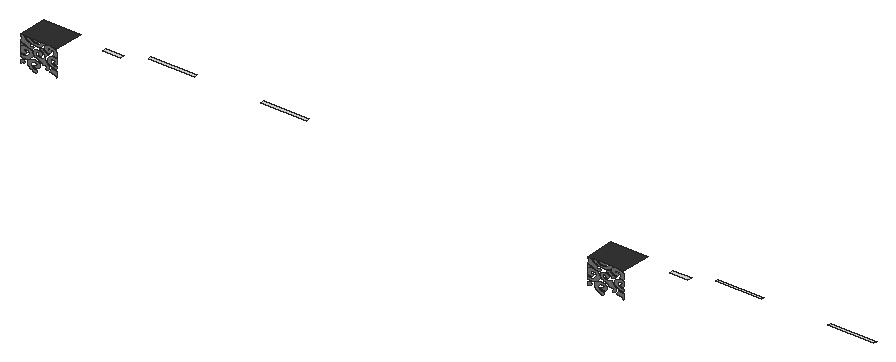
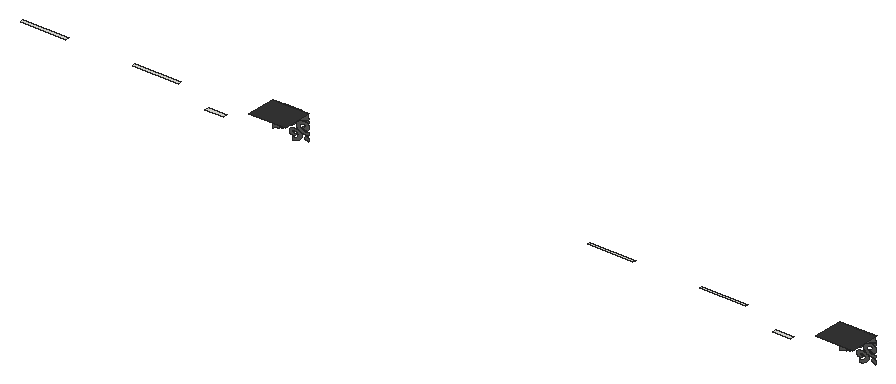
# SketchUp Ruby script. Lengths in inches.
U = 1.inch
M = Sketchup.active_model
def pt(a) = Geom::Point3d.new(a.map { |v| v * U })
def face(e, loops, mat)
  f = e.add_face(loops[0].map { |a| pt(a) })
  loops[1..].each { |l| e.add_face(l.map { |a| pt(a) }).erase! }
  f.material = f.back_material = mat if mat
  f
end
# faces: each face lists its corners as indices into pts; further lists are holes
def faces(e, pts, list, mat = nil) = list.each { |f| face(e, (f[0].is_a?(Array) ? f : [f]).map { |l| l.map { |i| pts[i] } }, mat) }
# xy, xz, yz: faces in a plane at the given z, y or x. An outline is a flat list of corners, or four numbers for a rectangle; further outlines are holes
def ring(l) = l.size == 4 ? [[l[0], l[1]], [l[2], l[1]], [l[2], l[3]], [l[0], l[3]]] : l.each_slice(2).to_a
def flat(e, list, mat, &to3) = list.each { |f| face(e, (f[0].is_a?(Array) ? f : [f]).map { |l| ring(l).map { |u, v| to3.(u, v) } }, mat) }
def xy(e, z, list, mat = nil) = flat(e, list, mat) { |x, y| [x, y, z] }
def xz(e, y, list, mat = nil) = flat(e, list, mat) { |x, z| [x, y, z] }
def yz(e, x, list, mat = nil) = flat(e, list, mat) { |y, z| [x, y, z] }
def lines(e, pts, list) = list.each { |a, b| e.add_line(pt(pts[a]), pt(pts[b])) }
# prism: a flat outline (further loops are holes) pulled along v
def prism(e, loops, v, mat = nil)
  f = face(e, loops, mat); d = Geom::Vector3d.new(v.map { |x| x * U })
  f.pushpull(f.normal.samedirection?(d) ? d.length : -d.length)
end
def box(e, o, s, mat = nil) = prism(e, [[o, [o[0] + s[0], o[1], o[2]], [o[0] + s[0], o[1] + s[1], o[2]], [o[0], o[1] + s[1], o[2]]]], [0, 0, s[2]], mat)
def at(x, y, z, deg = 0) = Geom::Transformation.translation(pt([x, y, z])) * Geom::Transformation.rotation(ORIGIN, Z_AXIS, deg.degrees)
def axes(o, x, y, z) = Geom::Transformation.new([*x, 0, *y, 0, *z, 0, *pt(o).to_a, 1])
def part(name) = M.definitions.add(name)
# library, detail: a bought-in or finely detailed component or shape, given as its bounding box
def library(name, o, s) = part(name).tap { |d| box(d.entities, o, s) }
def detail(e, o, s) = box(e.add_group.entities, o, s)
def put(e, d, t, mat = nil) = e.add_instance(d, t).tap { |i| i.material = mat if mat }
def group(e, t, mat = nil) = e.add_group.tap { |g| g.transformation = t; g.material = mat if mat }.entities
root = M.entities
M.materials.add("[0043_SaddleBrown]4").color = [124, 123, 122]
M.materials.add("[Slate Light Tile]").color = [54, 54, 54]
xy(root,742.22,[[2997.35,656.57,3037.18,665.86],[4247.98,656.57,4287.81,665.86]])
xy(root,759.44,[[2869.23,589.17,2950.32,653.8],[4119.85,589.17,4200.95,653.8]],"[Slate Light Tile]")
xy(root,766.875,[[3103.26,651.03,3204.51,657.03],[3351.01,651.03,3452.26,657.03],[4353.89,651.03,4455.14,657.03],[4601.63,651.03,4702.88,657.03]])
xz(root,589.17,[[2903.96,695.68,2904.37,696.06,2904.73,696.46,2905.05,696.87,2905.31,697.3,2905.52,697.74,2905.67,698.18,2905.78,698.63,2905.82,699.09,2905.81,699.55,2905.74,700,2905.625,700.45,2905.45,700.89,2904.1,700.8,2902.74,700.82,2901.39,700.95,2900.09,701.2,2898.86,701.55,2897.72,702,2896.6875,702.55,2895.79,703.18,2895.05,703.88,2894.46,704.64,2894.06,705.43,2893.83,706.26,2893.47,707.04,2893.24,707.83,2893.15,708.64,2893.2,709.45,2893.39,710.26,2893.72,711.04,2894.19,711.8,2894.79,712.52,2895.5,713.2,2896.34,713.83,2897.28,714.4,2898.31,714.91,2899.26,715.25,2900.31,715.47,2901.4,715.57,2902.51,715.54,2903.58,715.38,2904.59,715.1,2905.49,714.71,2906.26,714.21,2906.86,713.64,2907.27,713.01,2907.49,712.35,2907.49,711.67,2907.4,711.33,2907.24,711.01,2907.01,710.7,2906.72,710.42,2906.36,710.16,2905.95,709.93,2905.49,709.74,2904.99,709.59,2904.47,709.49,2903.93,709.43,2903.375,709.41,2902.83,709.4375,2902.25,709.45,2901.6875,709.39,2901.16,709.25,2900.7,709.03,2900.34,708.76,2900.08,708.45,2899.94,708.11,2899.9375,707.75,2900.0625,707.41,2900.3125,707.09,2900.67,706.82,2901.125,706.6,2902.37,706.22,2903.71,705.99,2905.09,705.91,2906.48,705.99,2907.8125,706.22,2909.06,706.6,2910.18,707.11,2911.12,707.73,2911.87,708.45,2912.39,709.24,2912.67,710.08,2912.69,710.93,2912.75,711.96,2912.57,712.99,2912.17,713.99,2911.54,714.95,2910.71,715.85,2909.68,716.67,2908.48,717.39,2907.13,718.01,2905.66,718.51,2904.09,718.875,2902.45,719.11,2900.77,719.2,2898.4375,719.12,2896.15,718.81,2893.97,718.29,2891.95,717.5625,2890.14,716.65,2888.59,715.58,2887.32,714.375,2886.375,713.0625,2885.77,711.67,2885.54,710.24,2885.66,708.81,2886.15,707.4,2886.71,706.04,2887.46,704.71,2888.42,703.44,2889.56,702.22,2890.87,701.07,2892.35,699.99,2893.99,699.01,2895.77,698.125,2897.67,697.34,2899.68,696.67,2901.78,696.11],[4154.58,695.68,4154.99,696.06,4155.36,696.46,4155.67,696.87,4155.93,697.3,4156.14,697.74,4156.3,698.18,4156.4,698.63,4156.45,699.09,4156.44,699.55,4156.37,700,4156.25,700.45,4156.07,700.89,4154.72,700.8,4153.36,700.82,4152.02,700.95,4150.72,701.2,4149.48,701.55,4148.34,702,4147.3125,702.55,4146.42,703.18,4145.67,703.88,4145.09,704.64,4144.68,705.43,4144.46,706.26,4144.09,707.04,4143.86,707.83,4143.77,708.64,4143.82,709.45,4144.02,710.26,4144.35,711.04,4144.81,711.8,4145.41,712.52,4146.13,713.2,4146.96,713.83,4147.9,714.4,4148.93,714.91,4149.89,715.25,4150.93,715.47,4152.03,715.57,4153.13,715.54,4154.21,715.38,4155.22,715.1,4156.12,714.71,4156.88,714.21,4157.49,713.64,4157.9,713.01,4158.11,712.35,4158.12,711.67,4158.03,711.33,4157.87,711.01,4157.64,710.7,4157.34,710.42,4156.98,710.16,4156.57,709.93,4156.11,709.74,4155.62,709.59,4155.1,709.49,4154.55,709.43,4154,709.41,4153.45,709.4375,4152.88,709.45,4152.3125,709.39,4151.79,709.25,4151.33,709.03,4150.96,708.76,4150.7,708.45,4150.57,708.11,4150.5625,707.75,4150.6875,707.41,4150.9375,707.09,4151.3,706.82,4151.75,706.6,4153,706.22,4154.33,705.99,4155.72,705.91,4157.1,705.99,4158.4375,706.22,4159.69,706.6,4160.8,707.11,4161.75,707.73,4162.49,708.45,4163.01,709.24,4163.29,710.08,4163.32,710.93,4163.37,711.96,4163.2,712.99,4162.79,713.99,4162.17,714.95,4161.33,715.85,4160.31,716.67,4159.11,717.39,4157.76,718.01,4156.28,718.51,4154.71,718.875,4153.07,719.11,4151.4,719.2,4149.0625,719.12,4146.78,718.81,4144.6,718.29,4142.58,717.5625,4140.77,716.65,4139.21,715.58,4137.94,714.375,4137,713.0625,4136.4,711.67,4136.16,710.24,4136.29,708.81,4136.78,707.4,4137.33,706.04,4138.09,704.71,4139.04,703.44,4140.18,702.22,4141.5,701.07,4142.98,699.99,4144.62,699.01,4146.39,698.125,4148.29,697.34,4150.3,696.67,4152.41,696.11],[2950.32,702.875,2950.32,713.56,2949.28,713.58,2948.25,713.62,2947.21,713.6875,2946.1875,713.78,2945.17,713.9,2944.15,714.04,2943.15,714.21,2942.16,714.4,2941.18,714.62,2940.22,714.85,2939.27,715.12,2938.34,715.4,2938.24,714.74,2938.08,714.08,2937.87,713.43,2937.6,712.78,2937.28,712.15,2936.91,711.52,2936.48,710.91,2936.01,710.3125,2935.49,709.73,2934.92,709.16,2934.3,708.61,2933.64,708.09,2935.29,708.18,2936.95,708.17,2938.6,708.05,2940.23,707.83,2941.8,707.51,2943.32,707.1,2944.76,706.59,2946.11,705.99,2947.35,705.32,2948.48,704.57,2949.47,703.75],[4200.95,702.875,4200.95,713.56,4199.91,713.58,4198.87,713.62,4197.84,713.6875,4196.8125,713.78,4195.79,713.9,4194.78,714.04,4193.78,714.21,4192.78,714.4,4191.81,714.62,4190.84,714.85,4189.9,715.12,4188.97,715.4,4188.86,714.74,4188.7,714.08,4188.49,713.43,4188.22,712.78,4187.9,712.15,4187.53,711.52,4187.11,710.91,4186.63,710.3125,4186.11,709.73,4185.54,709.16,4184.93,708.61,4184.26,708.09,4185.92,708.18,4187.58,708.17,4189.23,708.05,4190.85,707.83,4192.43,707.51,4193.95,707.1,4195.39,706.59,4196.73,705.99,4197.98,705.32,4199.1,704.57,4200.09,703.75],[2869.93,702.96,2870.45,703.5,2871.04,704.02,2871.7,704.5,2872.42,704.95,2873.19,705.36,2874.02,705.73,2874.9,706.0625,2875.8125,706.35,2876.76,706.58,2877.74,706.77,2878.74,706.91,2879.76,707,2879.34,707.42,2878.96,707.85,2878.61,708.29,2878.3,708.74,2878.03,709.2,2877.8,709.67,2877.61,710.15,2877.46,710.63,2877.36,711.12,2877.29,711.61,2877.26,712.1,2877.28,712.59,2876.58,712.37,2875.89,712.13,2875.22,711.88,2874.56,711.62,2873.92,711.34,2873.3,711.04,2872.69,710.74,2872.1,710.42,2871.53,710.09,2870.98,709.75,2870.44,709.39,2869.93,709.02],
  [4120.56,702.96,4121.08,703.5,4121.67,704.02,4122.32,704.5,4123.04,704.95,4123.82,705.36,4124.65,705.73,4125.52,706.0625,4126.4375,706.35,4127.39,706.58,4128.37,706.77,4129.37,706.91,4130.38,707,4129.96,707.42,4129.58,707.85,4129.24,708.29,4128.93,708.74,4128.66,709.2,4128.43,709.67,4128.24,710.15,4128.09,710.63,4127.98,711.12,4127.91,711.61,4127.89,712.1,4127.9,712.59,4127.2,712.37,4126.52,712.13,4125.85,711.88,4125.19,711.62,4124.55,711.34,4123.92,711.04,4123.32,710.74,4122.73,710.42,4122.15,710.09,4121.6,709.75,4121.07,709.39,4120.56,709.02],[2928.01,710.37,2928.57,710.4,2929.11,710.47,2929.63,710.59,2930.12,710.76,2930.57,710.97,2930.96,711.21,2931.29,711.49,2931.56,711.79,2931.75,712.11,2931.86,712.44,2931.9,712.79,2932.11,713.36,2932.26,713.9375,2932.34,714.52,2932.34,715.1,2932.28,715.6875,2932.15,716.27,2931.95,716.84,2931.68,717.4,2931.35,717.95,2930.95,718.49,2930.49,719,2929.97,719.49,2929.04,720.35,2928.17,721.23,2927.36,722.14,2926.625,723.07,2925.96,724.02,2925.36,724.99,2924.84,725.97,2924.39,726.97,2924.01,727.97,2923.71,728.99,2923.48,730.01,2923.33,731.04,2922.36,730.28,2921.24,729.6,2919.99,729.01,2918.62,728.53,2917.16,728.17,2915.64,727.92,2914.08,727.8,2912.5,727.8,2910.9375,727.93,2909.42,728.18,2907.96,728.55,2906.6,729.04,2905.625,729.5,2904.76,730.03,2904.01,730.625,2903.39,731.27,2902.91,731.97,2902.58,732.69,2902.41,733.4375,2902.39,734.19,2902.53,734.94,2902.83,735.67,2903.28,736.37,2903.87,737.03,2904.41,737.29,2905.01,737.48,2905.66,737.625,2906.33,737.71,2907.01,737.73,2907.6875,737.68,2908.35,737.58,2908.98,737.41,2909.56,737.19,2910.08,736.92,2910.53,736.6,2910.89,736.25,2910.77,736,2910.6875,735.74,2910.63,735.48,2910.61,735.22,2910.63,734.96,2910.68,734.7,2910.76,734.44,2910.87,734.1875,2911.02,733.94,2911.19,733.7,2911.4,733.48,2911.64,733.26,2911.87,733.09,2912.14,732.95,2912.45,732.83,2912.78,732.75,2913.13,732.7,2913.49,732.68,2913.84,732.7,2914.19,732.75,2914.52,732.83,2914.83,732.95,2915.1,733.09,2915.33,733.26,2916.01,733.94,2916.48,734.69,2916.74,735.48,2916.77,736.28,2916.58,737.07,2916.17,737.83,2915.5625,738.54,2914.76,739.18,2913.8,739.72,2912.7,740.15,2911.49,740.46,2910.22,740.63,2908.8,740.79,2907.36,740.82,2905.92,740.71,2904.53,740.47,2903.22,740.1,2902.01,739.62,2900.9375,739.02,2900.02,738.34,2899.29,737.58,2898.75,736.75,2898.42,735.89,2898.3125,735,2898.2,733.98,2898.26,732.96,2898.5,731.95,2898.9,730.96,2899.47,730,2900.2,729.08,2901.08,728.21,2902.1,727.4,2903.25,726.66,2904.52,726,2905.89,725.42,2907.35,724.9375,2908.74,724.49,2910.08,723.99,2911.35,723.43,2912.55,722.82,2913.68,722.15,2914.74,721.44,2915.7,720.68,2916.58,719.89,2917.36,719.05,2918.04,718.19,2918.63,717.3,2919.11,716.38,2919.78,716.7,2920.52,716.95,2921.32,717.14,2922.14,717.27,2922.99,717.32,2923.84,717.31,2924.67,717.22,2925.49,717.0625,2926.25,716.84,2926.97,716.55,2927.61,716.21,2928.17,715.82,2928.38,715.51,2928.53,715.18,2928.61,714.84,2928.63,714.5,2928.59,714.16,2928.49,713.83,2928.33,713.5,2928.11,713.1875,2927.83,712.89,2927.5,712.62,2927.125,712.37,2926.7,712.15,2926.47,712.02,2926.29,711.86,2926.16,711.6875,2926.09,711.5,2926.08,711.31,2926.125,711.12,2926.23,710.9375,2926.4,710.77,2926.61,710.63,2926.86,710.52,2927.15,710.4375,2927.45,710.39],[4178.63,710.37,4179.19,710.4,4179.74,710.47,4180.26,710.59,4180.75,710.76,4181.19,710.97,4181.58,711.21,4181.92,711.49,4182.18,711.79,4182.37,712.11,4182.49,712.44,4182.52,712.79,4182.74,713.36,4182.88,713.9375,4182.96,714.52,4182.97,715.1,4182.91,715.6875,4182.77,716.27,4182.57,716.84,4182.31,717.4,4181.97,717.95,4181.58,718.49,4181.12,719,4180.6,719.49,4179.66,720.35,4178.79,721.23,4177.99,722.14,4177.25,723.07,4176.58,724.02,4175.99,724.99,4175.46,725.97,4175.01,726.97,4174.63,727.97,4174.33,728.99,4174.11,730.01,4173.95,731.04,4172.99,730.28,4171.87,729.6,4170.61,729.01,4169.24,728.53,4167.79,728.17,4166.26,727.92,4164.7,727.8,4163.125,727.8,4161.5625,727.93,4160.04,728.18,4158.59,728.55,4157.22,729.04,4156.25,729.5,4155.38,730.03,4154.63,730.625,4154.01,731.27,4153.54,731.97,4153.21,732.69,4153.03,733.4375,4153.02,734.19,4153.16,734.94,4153.45,735.67,4153.9,736.37,4154.49,737.03,4155.04,737.29,4155.64,737.48,4156.28,737.625,4156.95,737.71,4157.63,737.73,4158.3125,737.68,4158.97,737.58,4159.6,737.41,4160.18,737.19,4160.7,736.92,4161.15,736.6,4161.52,736.25,4161.4,736,4161.3125,735.74,4161.26,735.48,4161.24,735.22,4161.25,734.96,4161.3,734.7,4161.38,734.44,4161.5,734.1875,4161.64,733.94,4161.82,733.7,4162.03,733.48,4162.26,733.26,4162.5,733.09,4162.77,732.95,4163.07,732.83,4163.41,732.75,4163.75,732.7,4164.11,732.68,4164.47,732.7,4164.82,732.75,4165.15,732.83,4165.45,732.95,4165.73,733.09,4165.96,733.26,4166.63,733.94,4167.1,734.69,4167.36,735.48,4167.4,736.28,4167.21,737.07,4166.8,737.83,4166.1875,738.54,4165.39,739.18,4164.42,739.72,4163.32,740.15,4162.12,740.46,4160.84,740.63,4159.42,740.79,4157.98,740.82,4156.55,740.71,4155.16,740.47,4153.84,740.1,4152.64,739.62,4151.5625,739.02,4150.65,738.34,4149.91,737.58,4149.375,736.75,4149.05,735.89,4148.9375,735,4148.83,733.98,4148.89,732.96,4149.12,731.95,4149.53,730.96,4150.09,730,4150.82,729.08,4151.7,728.21,4152.72,727.4,4153.87,726.66,4155.14,726,4156.52,725.42,4157.98,724.9375,4159.37,724.49,4160.7,723.99,4161.97,723.43,4163.18,722.82,4164.31,722.15,4165.36,721.44,4166.33,720.68,4167.2,719.89,4167.99,719.05,4168.67,718.19,4169.25,717.3,4169.73,716.38,4170.41,716.7,4171.15,716.95,4171.94,717.14,4172.77,717.27,4173.61,717.32,4174.46,717.31,4175.3,717.22,4176.11,717.0625,4176.88,716.84,4177.59,716.55,4178.24,716.21,4178.8,715.82,4179,715.51,4179.15,715.18,4179.24,714.84,4179.26,714.5,4179.22,714.16,4179.12,713.83,4178.95,713.5,4178.73,713.1875,4178.46,712.89,4178.125,712.62,4177.75,712.37,4177.33,712.15,4177.1,712.02,4176.91,711.86,4176.78,711.6875,4176.71,711.5,4176.7,711.31,4176.75,711.12,4176.86,710.9375,4177.02,710.77,4177.24,710.63,4177.49,710.52,4177.77,710.4375,4178.08,710.39],[2876.55,715.57,2878.81,715.62,2881.04,715.84,2883.22,716.22,2885.3,716.76,2887.27,717.44,2889.09,718.27,2890.73,719.23,2892.18,720.29,2893.41,721.46,2895.07,723.2,2896.23,725.09,2896.84,727.07,2896.89,729.09,2896.37,731.08,2895.3,732.99,2893.7,734.75,2891.64,736.33,2889.17,737.66,2886.36,738.7,2883.3,739.44,2880.08,739.84,2878.93,739.71,2877.79,739.5,2876.7,739.24,2875.65,738.91,2874.65,738.52,2873.72,738.07,2872.87,737.57,2872.09,737.02,2871.4,736.43,2870.8125,735.81,2870.32,735.15,2869.93,734.46,2869.93,727.58,2870.46,726.8,2871.24,726.12,2872.23,725.54,2873.38,725.1,2874.66,724.81,2876.01,724.6875,2877.37,724.74,2878.6875,724.95,2879.91,725.33,2880.97,725.85,2881.84,726.5,2882.48,727.24,2882.57,727.41,2882.625,727.6,2882.63,727.79,2882.59,727.97,2882.51,728.15,2882.38,728.32,2882.22,728.48,2882.01,728.62,2881.78,728.74,2881.52,728.84,2881.24,728.91,2880.95,728.96,2880.22,728.89,2879.49,728.89,2878.76,728.98,2878.08,729.15,2877.46,729.4,2876.92,729.71,2876.49,730.08,2876.17,730.48,2875.99,730.92,2875.93,731.375,2876.01,731.82,2876.23,732.26,2876.41,732.82,2876.74,733.36,2877.19,733.86,2877.77,734.3,2878.46,734.69,2879.24,735.01,2880.09,735.24,2880.99,735.4,2881.92,735.46,2882.85,735.43,2883.76,735.3125,2884.64,735.11,2885.99,734.44,2887.18,733.66,2888.18,732.78,2888.96,731.83,2889.52,730.81,2889.84,729.76,2889.91,728.7,2889.74,727.63,2889.32,726.59,2888.67,725.6,2887.79,724.68,2886.72,723.84,2886.28,723.28,2885.76,722.75,2885.18,722.25,2884.53,721.77,2883.82,721.34,2883.06,720.9375,2882.24,720.58,2881.37,720.26,2880.47,719.99,2879.53,719.77,2878.57,719.59,2877.58,719.47,2876.88,719.42,2876.17,719.4,2875.47,719.42,2874.77,719.48,2874.08,719.58,2873.4,719.7,2872.75,719.87,2872.12,720.0625,2871.52,720.29,2870.95,720.55,2870.42,720.84,2869.93,721.15,2869.93,716.4,2872.08,715.96,2874.29,715.68],[4127.17,715.57,4129.43,715.62,4131.67,715.84,4133.84,716.22,4135.93,716.76,4137.89,717.44,4139.71,718.27,4141.36,719.23,4142.8,720.29,4144.03,721.46,4145.7,723.2,4146.86,725.09,4147.47,727.07,4147.51,729.09,4146.99,731.08,4145.92,732.99,4144.33,734.75,4142.27,736.33,4139.8,737.66,4136.99,738.7,4133.93,739.44,4130.71,739.84,4129.55,739.71,4128.42,739.5,4127.32,739.24,4126.27,738.91,4125.28,738.52,4124.35,738.07,4123.49,737.57,4122.72,737.02,4122.03,736.43,4121.4375,735.81,4120.95,735.15,4120.56,734.46,4120.56,727.58,4121.09,726.8,4121.86,726.12,4122.85,725.54,4124.01,725.1,4125.29,724.81,4126.64,724.6875,4128,724.74,4129.3125,724.95,4130.53,725.33,4131.6,725.85,4132.47,726.5,4133.11,727.24,4133.2,727.41,4133.25,727.6,4133.25,727.79,4133.22,727.97,4133.13,728.15,4133.01,728.32,4132.84,728.48,4132.64,728.62,4132.41,728.74,4132.15,728.84,4131.87,728.91,4131.57,728.96,4130.85,728.89,4130.11,728.89,4129.39,728.98,4128.71,729.15,4128.09,729.4,4127.55,729.71,4127.12,730.08,4126.8,730.48,4126.61,730.92,4126.56,731.375,4126.64,731.82,4126.85,732.26,4127.04,732.82,4127.36,733.36,4127.82,733.86,4128.4,734.3,4129.09,734.69,4129.87,735.01,4130.72,735.24,4131.62,735.4,4132.54,735.46,4133.48,735.43,4134.39,735.3125,4135.26,735.11,4136.62,734.44,4137.81,733.66,4138.8,732.78,4139.59,731.83,4140.14,730.81,4140.46,729.76,4140.53,728.7,4140.36,727.63,4139.94,726.59,4139.29,725.6,4138.42,724.68,4137.34,723.84,4136.9,723.28,4136.39,722.75,4135.81,722.25,4135.16,721.77,4134.45,721.34,4133.68,720.9375,4132.86,720.58,4132,720.26,4131.09,719.99,4130.16,719.77,4129.19,719.59,4128.21,719.47,4127.5,719.42,4126.8,719.4,4126.09,719.42,4125.39,719.48,4124.7,719.58,4124.03,719.7,4123.375,719.87,4122.74,720.0625,4122.14,720.29,4121.58,720.55,4121.05,720.84,4120.56,721.15,4120.56,716.4,4122.7,715.96,4124.92,715.68],
  [2947.73,718.47,2950.32,718.69,2950.32,722.69,2948.09,722.65,2945.88,722.84,2943.76,723.27,2941.79,723.91,2940.04,724.76,2938.55,725.78,2937.37,726.94,2936.54,728.21,2936.08,729.55,2936.01,730.92,2936.32,732.28,2937.02,733.58,2937.8125,734.14,2938.77,734.59,2939.84,734.93,2941,735.14,2942.2,735.21,2943.4,735.13,2944.56,734.93,2945.63,734.59,2946.58,734.13,2947.375,733.57,2947.98,732.93,2948.38,732.23,2948.46,731.95,2948.45,731.66,2948.36,731.375,2948.2,731.11,2947.96,730.86,2947.66,730.64,2947.3,730.46,2946.9,730.3125,2946.46,730.21,2946,730.16,2945.53,730.16,2945.07,730.2,2944.82,730.14,2944.6,730.06,2944.38,729.96,2944.1875,729.85,2944.01,729.73,2943.86,729.6,2943.73,729.45,2943.63,729.3,2943.55,729.15,2943.51,728.99,2943.49,728.83,2943.49,728.67,2943.86,728.34,2944.3,728.04,2944.8,727.78,2945.35,727.5625,2945.9375,727.39,2946.56,727.27,2947.2,727.2,2947.85,727.1875,2948.5,727.22,2949.14,727.3125,2949.75,727.45,2950.32,727.64,2950.32,737.55,2949.26,738.08,2948.11,738.51,2946.87,738.86,2945.57,739.11,2944.24,739.26,2942.88,739.32,2941.53,739.26,2940.19,739.11,2938.9,738.86,2937.66,738.51,2936.5,738.08,2935.44,737.55,2934.55,737.02,2933.72,736.46,2932.94,735.86,2932.24,735.23,2931.61,734.57,2931.05,733.89,2930.57,733.18,2930.16,732.46,2929.83,731.72,2929.59,730.97,2929.43,730.22,2929.35,729.45,2929.46,727.85,2929.97,726.27,2930.86,724.75,2932.11,723.34,2933.69,722.06,2935.57,720.94,2937.7,720,2940.04,719.27,2942.52,718.77,2945.11,718.5],[4198.35,718.47,4200.95,718.69,4200.95,722.69,4198.72,722.65,4196.51,722.84,4194.39,723.27,4192.42,723.91,4190.66,724.76,4189.17,725.78,4188,726.94,4187.16,728.21,4186.7,729.55,4186.63,730.92,4186.95,732.28,4187.64,733.58,4188.4375,734.14,4189.39,734.59,4190.47,734.93,4191.625,735.14,4192.83,735.21,4194.03,735.13,4195.19,734.93,4196.26,734.59,4197.21,734.13,4198,733.57,4198.61,732.93,4199.01,732.23,4199.08,731.95,4199.07,731.66,4198.99,731.375,4198.82,731.11,4198.59,730.86,4198.28,730.64,4197.93,730.46,4197.52,730.3125,4197.08,730.21,4196.62,730.16,4196.15,730.16,4195.69,730.2,4195.45,730.14,4195.22,730.06,4195.01,729.96,4194.8125,729.85,4194.64,729.73,4194.49,729.6,4194.36,729.45,4194.26,729.3,4194.18,729.15,4194.13,728.99,4194.11,728.83,4194.12,728.67,4194.49,728.34,4194.92,728.04,4195.42,727.78,4195.97,727.5625,4196.5625,727.39,4197.18,727.27,4197.82,727.2,4198.48,727.1875,4199.125,727.22,4199.76,727.3125,4200.37,727.45,4200.95,727.64,4200.95,737.55,4199.89,738.08,4198.73,738.51,4197.49,738.86,4196.2,739.11,4194.86,739.26,4193.51,739.32,4192.15,739.26,4190.82,739.11,4189.52,738.86,4188.29,738.51,4187.13,738.08,4186.07,737.55,4185.17,737.02,4184.34,736.46,4183.57,735.86,4182.87,735.23,4182.23,734.57,4181.67,733.89,4181.19,733.18,4180.79,732.46,4180.46,731.72,4180.21,730.97,4180.05,730.22,4179.97,729.45,4180.09,727.85,4180.6,726.27,4181.49,724.75,4182.74,723.34,4184.32,722.06,4186.19,720.94,4188.33,720,4190.66,719.27,4193.15,718.77,4195.73,718.5],[2924.43,735.95,2924.98,736.35,2925.54,736.73,2926.11,737.11,2926.69,737.49,2927.29,737.86,2927.89,738.22,2928.5,738.57,2929.12,738.93,2930.38,739.61,2931.03,739.94,2931.6875,740.26,2930.03,740.53,2928.42,740.9,2926.875,741.37,2925.41,741.92,2924.05,742.5625,2922.79,743.28,2921.65,744.07,2920.65,744.93,2919.79,745.84,2919.08,746.8,2918.52,747.8,2918.13,748.83,2917.65,748.48,2917.14,748.14,2916.62,747.82,2916.08,747.5,2915.52,747.2,2914.94,746.92,2914.34,746.64,2913.73,746.38,2913.11,746.13,2912.47,745.9,2911.81,745.68,2911.14,745.48,2912.71,744.99,2914.21,744.43,2915.64,743.8125,2917,743.13,2918.28,742.39,2919.47,741.6,2920.5625,740.76,2921.55,739.87,2922.44,738.94,2923.22,737.98,2923.88,736.98],[4175.05,735.95,4175.6,736.35,4176.74,737.11,4177.32,737.49,4177.91,737.86,4178.51,738.22,4179.12,738.57,4179.74,738.93,4180.37,739.27,4181.01,739.61,4181.66,739.94,4182.3125,740.26,4180.65,740.53,4179.04,740.9,4177.5,741.37,4176.04,741.92,4174.67,742.5625,4173.41,743.28,4172.28,744.07,4171.28,744.93,4170.41,745.84,4169.7,746.8,4169.15,747.8,4168.75,748.83,4168.27,748.48,4167.77,748.14,4167.25,747.82,4166.7,747.5,4166.14,747.2,4165.56,746.92,4164.97,746.64,4164.36,746.38,4163.73,746.13,4163.09,745.9,4162.44,745.68,4161.77,745.48,4163.33,744.99,4164.83,744.43,4166.27,743.8125,4167.63,743.13,4168.91,742.39,4170.09,741.6,4171.1875,740.76,4172.18,739.87,4173.07,738.94,4173.84,737.98,4174.51,736.98],[2869.93,739.1,2870.35,739.38,2870.79,739.65,2871.24,739.92,2871.71,740.16,2872.21,740.4,2872.71,740.62,2873.24,740.83,2873.77,741.02,2874.33,741.2,2874.89,741.36,2875.46,741.51,2876.05,741.64,2875.67,741.93,2875.26,742.19,2874.82,742.4375,2874.35,742.66,2873.86,742.87,2873.34,743.06,2872.81,743.22,2872.26,743.36,2871.6875,743.47,2871.11,743.5625,2870.53,743.63,2869.93,743.67],
  [4120.56,739.1,4120.97,739.38,4121.41,739.65,4121.87,739.92,4122.34,740.16,4122.83,740.4,4123.34,740.62,4123.86,740.83,4124.4,741.02,4124.95,741.2,4125.51,741.36,4126.09,741.51,4126.67,741.64,4126.29,741.93,4125.88,742.19,4125.44,742.4375,4124.97,742.66,4124.48,742.87,4123.97,743.06,4123.43,743.22,4122.88,743.36,4122.3125,743.47,4121.74,743.5625,4121.15,743.63,4120.56,743.67],[2891.98,739.72,2892.91,739.75,2893.81,739.85,2894.7,740,2895.56,740.21,2895.86,740.31,2896.15,740.42,2896.43,740.55,2896.68,740.6875,2896.92,740.84,2897.13,741,2897.33,741.18,2897.49,741.36,2897.64,741.55,2897.75,741.75,2897.84,741.95,2897.9,742.16,2897.92,742.37,2897.91,742.57,2897.86,742.77,2897.77,742.97,2897.65,743.16,2897.49,743.34,2897.3,743.51,2897.08,743.66,2896.83,743.8,2896.5625,743.92,2896.27,744.02,2895.96,744.09,2895.77,743.88,2895.35,743.48,2895.12,743.28,2894.88,743.09,2894.63,742.9,2894.375,742.72,2894.1,742.54,2893.83,742.375,2893.54,742.21,2893.24,742.05,2892.93,741.9,2892.51,741.96,2892.09,742.04,2891.69,742.15,2891.31,742.28,2890.96,742.43,2890.625,742.6,2890.32,742.79,2890.05,743,2889.8125,743.23,2889.61,743.46,2889.45,743.71,2889.33,743.97,2889.19,744.37,2889.08,744.78,2889,745.18,2888.95,745.6,2888.94,746.01,2888.96,746.42,2889.02,746.83,2889.11,747.24,2889.22,747.64,2889.375,748.04,2889.56,748.4375,2889.77,748.83,2888.31,749.17,2886.89,749.6,2885.55,750.09,2884.28,750.66,2883.1,751.3,2882.01,752,2881.03,752.76,2880.17,753.5625,2879.43,754.41,2878.81,755.3,2878.32,756.22,2877.97,757.16,2877.59,757.31,2877.21,757.47,2876.85,757.63,2876.49,757.81,2876.14,757.99,2875.81,758.17,2875.48,758.36,2875.16,758.5625,2874.85,758.77,2874.55,758.98,2874.26,759.19,2873.98,759.44,2869.93,759.44,2869.93,758.69,2871.02,757.9375,2871.9375,757.1,2872.67,756.2,2873.2,755.24,2873.52,754.26,2873.625,753.25,2873.52,752.24,2873.2,751.25,2872.67,750.3,2871.9375,749.4,2871.02,748.56,2869.93,747.8,2869.93,746.79,2871.41,746.6,2872.86,746.36,2874.29,746.08,2875.69,745.74,2877.0625,745.36,2878.4,744.93,2879.69,744.46,2880.94,743.95,2882.14,743.39,2883.29,742.79,2884.39,742.16,2885.43,741.49,2886.08,741.09,2886.8,740.73,2887.57,740.43,2888.39,740.17,2889.26,739.97,2890.15,739.83,2891.0625,739.74],[4142.61,739.72,4143.53,739.75,4144.44,739.85,4145.33,740,4146.18,740.21,4146.49,740.31,4146.78,740.42,4147.05,740.55,4147.31,740.6875,4147.54,740.84,4147.76,741,4147.95,741.18,4148.12,741.36,4148.26,741.55,4148.375,741.75,4148.46,741.95,4148.52,742.16,4148.55,742.37,4148.54,742.57,4148.49,742.77,4148.4,742.97,4148.28,743.16,4148.12,743.34,4147.93,743.51,4147.71,743.66,4147.46,743.8,4147.1875,743.92,4146.9,744.02,4146.59,744.09,4146.39,743.88,4146.19,743.68,4145.75,743.28,4145.51,743.09,4145.26,742.9,4145,742.72,4144.73,742.54,4144.45,742.375,4144.16,742.21,4143.86,742.05,4143.56,741.9,4143.13,741.96,4142.72,742.04,4142.32,742.15,4141.94,742.28,4141.58,742.43,4141.25,742.6,4140.95,742.79,4140.68,743,4140.4375,743.23,4140.24,743.46,4140.07,743.71,4139.95,743.97,4139.81,744.37,4139.7,744.78,4139.625,745.18,4139.58,745.6,4139.57,746.01,4139.59,746.42,4139.64,746.83,4139.73,747.24,4139.85,747.64,4140,748.04,4140.18,748.4375,4140.4,748.83,4138.93,749.17,4137.52,749.6,4136.17,750.09,4134.9,750.66,4133.72,751.3,4132.64,752,4131.66,752.76,4130.79,753.5625,4130.05,754.41,4129.43,755.3,4128.94,756.22,4128.59,757.16,4128.21,757.31,4127.47,757.63,4126.77,757.99,4126.43,758.17,4126.1,758.36,4125.78,758.5625,4125.47,758.77,4125.17,758.98,4124.88,759.19,4124.6,759.44,4120.56,759.44,4120.56,758.69,4121.64,757.9375,4122.5625,757.1,4123.29,756.2,4123.82,755.24,4124.14,754.26,4124.25,753.25,4124.14,752.24,4123.82,751.25,4123.29,750.3,4122.5625,749.4,4121.64,748.56,4120.56,747.8,4120.56,746.79,4122.03,746.6,4123.48,746.36,4124.92,746.08,4126.32,745.74,4127.6875,745.36,4129.02,744.93,4130.32,744.46,4131.57,743.95,4132.77,743.39,4133.92,742.79,4135.01,742.16,4136.05,741.49,4136.7,741.09,4137.42,740.73,4138.2,740.43,4139.02,740.17,4139.88,739.97,4140.78,739.83,4141.6875,739.74],[2950.32,741.3,2950.32,748.98,2949.91,750.12,2949.32,751.22,2948.55,752.29,2947.63,753.3,2946.55,754.26,2945.32,755.15,2943.96,755.96,2942.48,756.6875,2940.89,757.32,2939.21,757.86,2937.46,758.3,2935.64,758.63,2933.97,758.68,2932.3125,758.58,2930.69,758.33,2929.15,757.93,2927.73,757.4,2926.45,756.74,2925.34,755.98,2924.43,755.12,2923.73,754.18,2923.27,753.2,2923.05,752.18,2923.08,751.16,2923.04,750.51,2923.12,749.86,2923.33,749.23,2923.66,748.61,2924.11,748.03,2924.68,747.48,2925.34,746.98,2926.11,746.53,2926.95,746.14,2927.87,745.82,2928.84,745.57,2929.86,745.39,2930.54,745.15,2931.27,744.97,2932.04,744.88,2932.83,744.87,2933.61,744.94,2934.36,745.09,2935.05,745.32,2935.67,745.62,2936.2,745.97,2936.625,746.38,2936.93,746.83,2937.11,747.3,2937.5,747.65,2937.8,748.03,2937.98,748.4375,2938.05,748.86,2938,749.29,2937.83,749.7,2937.54,750.08,2937.15,750.4375,2936.67,750.74,2936.11,750.99,2935.49,751.18,2934.83,751.3,2934.35,750.88,2934.1,750.68,2933.83,750.49,2933.55,750.3,2933.27,750.12,2932.97,749.9375,2932.67,749.77,2932.35,749.6,2932.03,749.44,2931.7,749.29,2931.36,749.15,2930.99,749.29,2930.64,749.46,2930.33,749.65,2930.05,749.86,2929.8125,750.09,2929.61,750.33,2929.46,750.58,2929.35,750.84,2929.29,751.11,2929.27,751.38,2929.31,751.65,2929.39,751.92,2929.67,752.45,2930.1,752.95,2930.65,753.4,2931.31,753.79,2932.06,754.11,2932.89,754.36,2933.77,754.51,2934.68,754.58,2935.59,754.56,2936.49,754.44,2937.34,754.24,2938.14,753.96,2939.55,753.26,2940.8,752.46,2941.86,751.55,2942.72,750.57,2943.35,749.53,2943.74,748.44,2943.89,747.33,2943.8,746.22,2943.46,745.125,2942.88,744.07,2942.08,743.07,2941.06,742.15,2941.85,742.26,2942.64,742.34,2943.4375,742.39,2944.24,742.4,2945.04,742.38,2945.84,742.32,2946.63,742.24,2947.41,742.11,2948.17,741.96,2948.91,741.77,2949.63,741.55],[4200.95,741.3,4200.95,748.98,4200.53,750.12,4199.94,751.22,4199.18,752.29,4198.25,753.3,4197.17,754.26,4195.95,755.15,4194.59,755.96,4193.11,756.6875,4191.52,757.32,4189.84,757.86,4188.08,758.3,4186.26,758.63,4184.6,758.68,4182.9375,758.58,4181.32,758.33,4179.78,757.93,4178.35,757.4,4177.07,756.74,4175.96,755.98,4175.05,755.12,4174.36,754.18,4173.9,753.2,4173.68,752.18,4173.71,751.16,4173.66,750.51,4173.74,749.86,4173.95,749.23,4174.28,748.61,4174.74,748.03,4175.3,747.48,4175.97,746.98,4176.73,746.53,4177.58,746.14,4178.5,745.82,4179.47,745.57,4180.49,745.39,4181.16,745.15,4181.9,744.97,4182.67,744.88,4183.46,744.87,4184.23,744.94,4184.98,745.09,4185.67,745.32,4186.3,745.62,4186.83,745.97,4187.25,746.38,4187.55,746.83,4187.73,747.3,4188.13,747.65,4188.43,748.03,4188.61,748.4375,4188.68,748.86,4188.62,749.29,4188.45,749.7,4188.17,750.08,4187.78,750.4375,4187.3,750.74,4186.74,750.99,4186.12,751.18,4185.45,751.3,4185.22,751.09,4184.98,750.88,4184.72,750.68,4184.46,750.49,4184.18,750.3,4183.89,750.12,4183.6,749.9375,4183.29,749.77,4182.98,749.6,4182.66,749.44,4182.32,749.29,4181.99,749.15,4181.61,749.29,4181.27,749.46,4180.95,749.65,4180.68,749.86,4180.4375,750.09,4180.24,750.33,4180.08,750.58,4179.98,750.84,4179.91,751.11,4179.9,751.38,4179.93,751.65,4180.01,751.92,4180.3,752.45,4180.72,752.95,4181.27,753.4,4181.93,753.79,4182.68,754.11,4183.51,754.36,4184.39,754.51,4185.3,754.58,4186.22,754.56,4187.11,754.44,4187.97,754.24,4188.76,753.96,4190.18,753.26,4191.43,752.46,4192.49,751.55,4193.34,750.57,4193.97,749.53,4194.37,748.44,4194.52,747.33,4194.42,746.22,4194.08,745.125,4193.51,744.07,4192.7,743.07,4191.69,742.15,4192.47,742.26,4193.26,742.34,4194.0625,742.39,4194.86,742.4,4195.67,742.38,4196.46,742.32,4197.25,742.24,4198.03,742.11,4198.79,741.96,4199.53,741.77,4200.25,741.55],
  [2903.17,748.82,2907.99,749.18,2912.55,750.2,2916.6,751.84,2919.9375,754.01,2922.37,756.6,2923.77,759.44,2917.61,759.44,2916.43,757.58,2914.625,755.92,2912.27,754.53,2909.49,753.48,2906.4,752.83,2903.16,752.61,2899.92,752.81,2896.82,753.45,2894.02,754.48,2891.65,755.85,2889.82,757.51,2888.61,759.44,2882.45,759.44,2883.88,756.52,2886.34,753.95,2889.7,751.79,2893.77,750.17,2898.34,749.16],[4153.79,748.82,4158.61,749.18,4163.17,750.2,4167.23,751.84,4170.5625,754.01,4172.99,756.6,4174.4,759.44,4168.24,759.44,4167.06,757.58,4165.25,755.92,4162.9,754.53,4160.11,753.48,4157.03,752.83,4153.79,752.61,4150.54,752.81,4147.45,753.45,4144.65,754.48,4142.27,755.85,4140.44,757.51,4139.23,759.44,4133.08,759.44,4134.51,756.52,4136.97,753.95,4140.32,751.79,4144.39,750.17,4148.96,749.16],[2903.48,756.12,2905.24,756.22,2906.94,756.52,2908.52,757.02,2909.92,757.6875,2911.08,758.51,2911.98,759.44,2894.98,759.44,2895.88,758.51,2897.05,757.6875,2898.44,757.02,2900.02,756.52,2901.72,756.22],[4154.11,756.12,4155.87,756.22,4157.57,756.52,4159.15,757.02,4160.54,757.6875,4161.71,758.51,4162.6,759.44,4145.61,759.44,4146.5,758.51,4147.67,757.6875,4149.07,757.02,4150.64,756.52,4152.34,756.22]],"[0043_SaddleBrown]4")
p = [[2933.23,589.17,696.8],[2933.14,589.17,696.34],[2869.93,589.17,746.79],[2869.93,589.17,743.67],[4183.85,589.17,696.8],[4183.77,589.17,696.34],
  [4120.56,589.17,746.79],[4120.56,589.17,743.67]]
lines(root,p,[[0,1],[2,3],[4,5],[6,7]])
